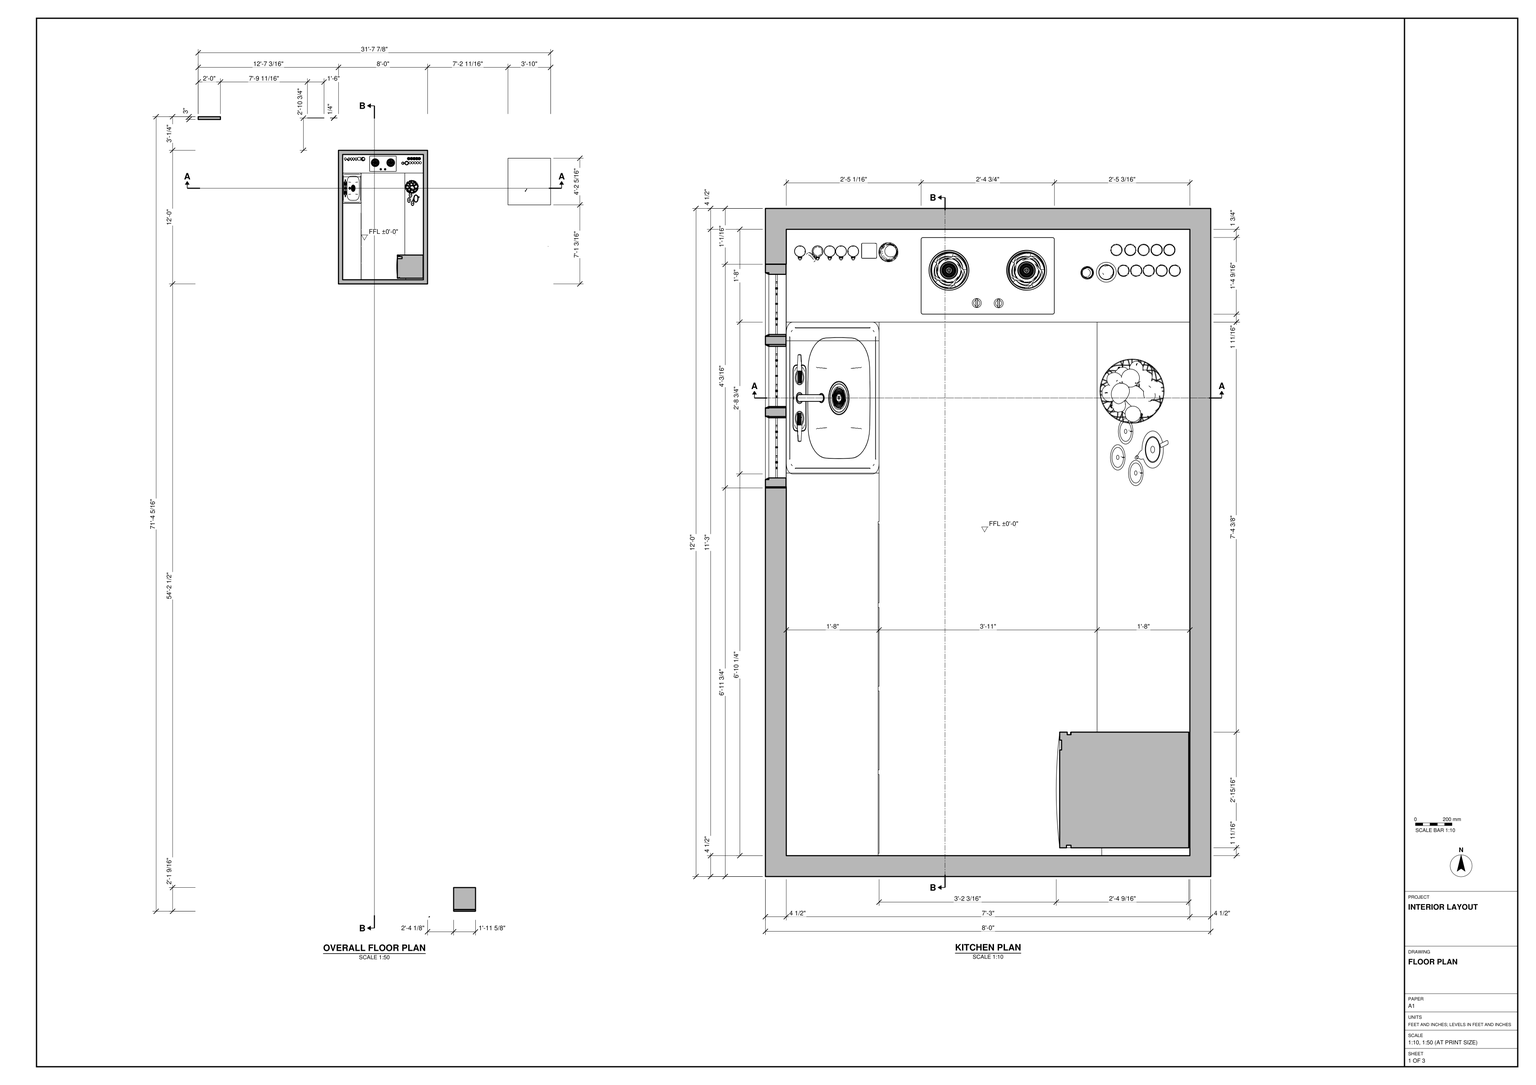
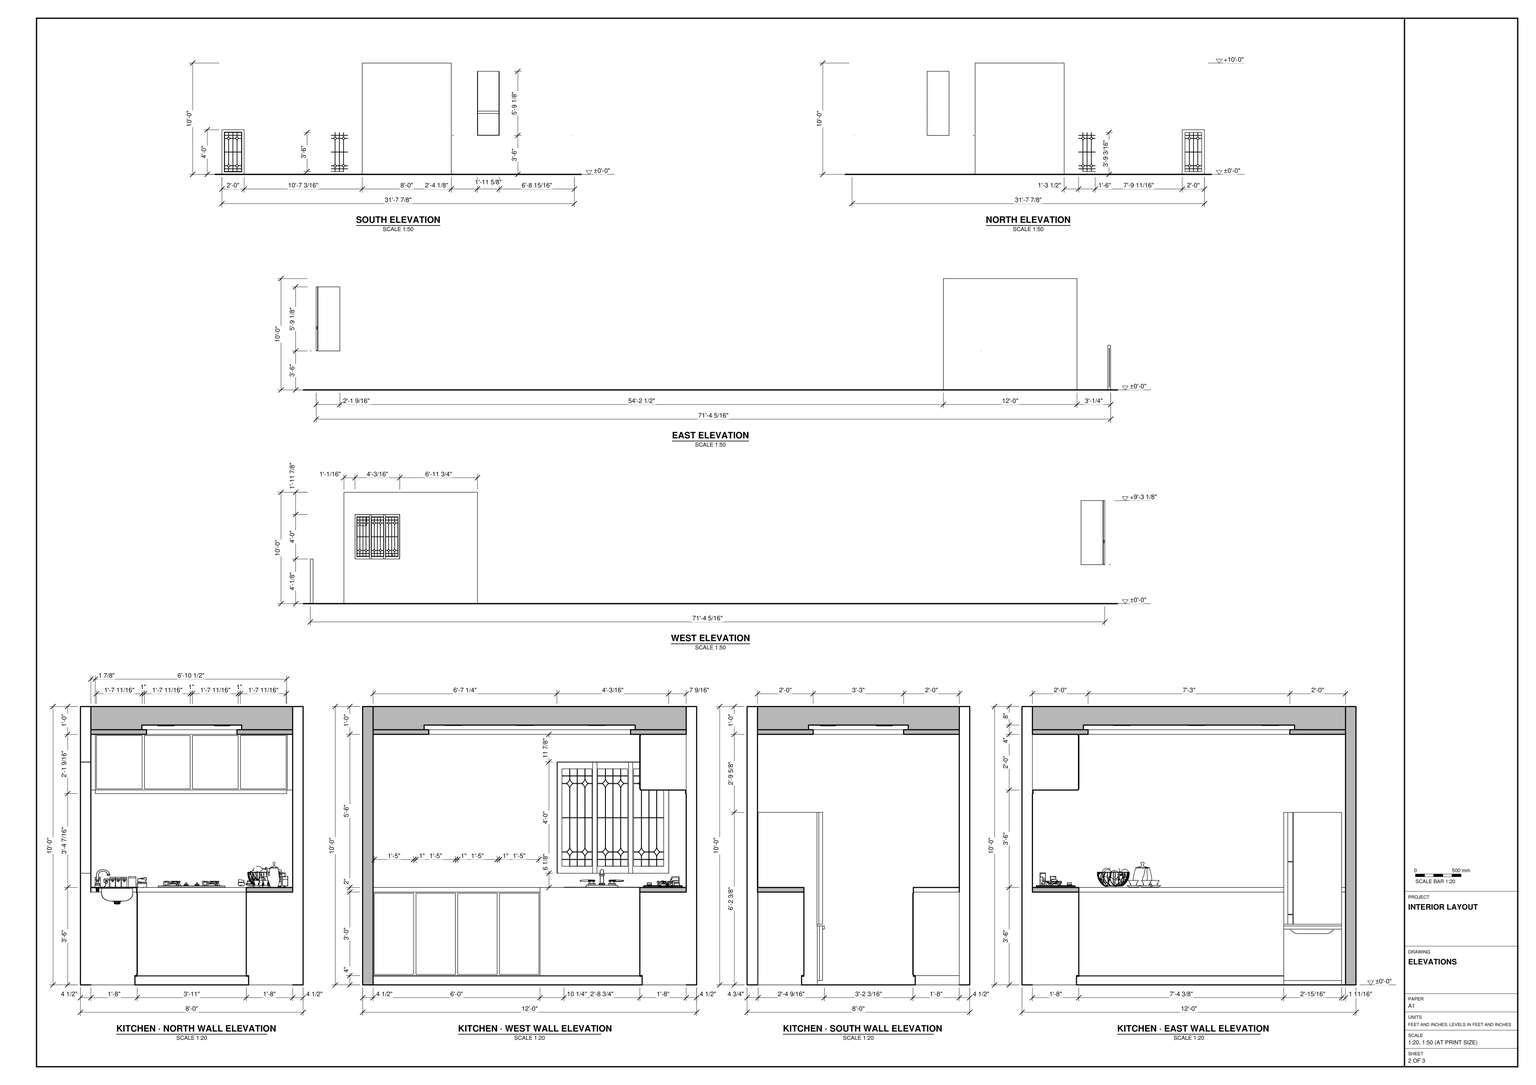
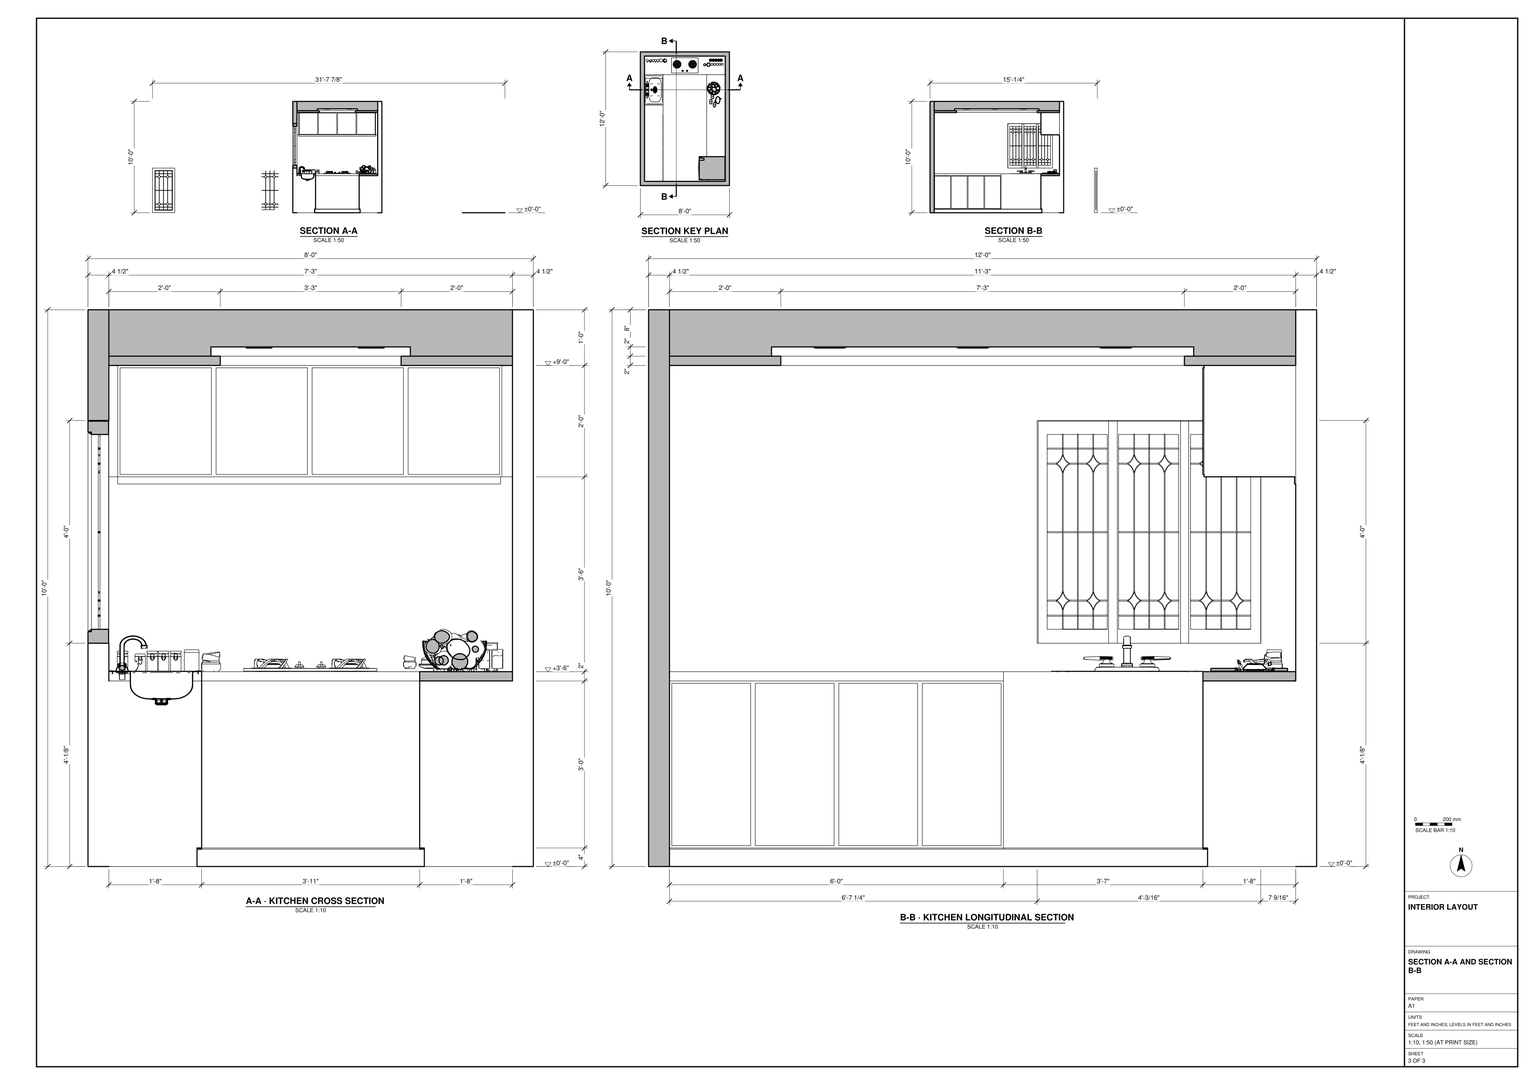
Build the kitchen in SketchUp from task_files/diagram_01.pdf. Work in feet and inches, with the finished floor at ±0'-0". Use the overall plan and elevations to position the kitchen and the detached elements outside it. The complete layout is 31'-7 7/8" wide by 71'-4 5/16" long and 10'-0" high; these are not the dimensions of the kitchen itself.

Model the kitchen shell at 8'-0" by 12'-0" externally, with 4 1/2" perimeter walls. Use the sections to form the floor and the stepped ceiling with its recessed central field. Fit the worktops along the north, west and east walls, leaving the central aisle clear. Follow the interior elevations for the extent and front divisions of the west base cabinets and the north wall cabinets. Set the sink and tap beneath the divided west window, place the cooktop on the north worktop and fit the refrigerator at the south end of the east run. Place the small countertop items in the areas indicated on the kitchen plan. Appliances, decor and loose items may be any suitable library components.

Keep shell elements and individual furniture or joinery pieces in separate groups or components, and use components for repeated parts. Save one SketchUp model as output_files/kitchen_interior_and_its_dimensioned_overall_layout.skp.

# SketchUp Ruby script. Lengths in inches.
U = 1.inch
M = Sketchup.active_model
def pt(a) = Geom::Point3d.new(a.map { |v| v * U })
def face(e, loops, mat)
  f = e.add_face(loops[0].map { |a| pt(a) })
  loops[1..].each { |l| e.add_face(l.map { |a| pt(a) }).erase! }
  f.material = f.back_material = mat if mat
  f
end
# faces: each face lists its corners as indices into pts; further lists are holes
def faces(e, pts, list, mat = nil) = list.each { |f| face(e, (f[0].is_a?(Array) ? f : [f]).map { |l| l.map { |i| pts[i] } }, mat) }
# xy, xz, yz: faces in a plane at the given z, y or x. An outline is a flat list of corners, or four numbers for a rectangle; further outlines are holes
def ring(l) = l.size == 4 ? [[l[0], l[1]], [l[2], l[1]], [l[2], l[3]], [l[0], l[3]]] : l.each_slice(2).to_a
def flat(e, list, mat, &to3) = list.each { |f| face(e, (f[0].is_a?(Array) ? f : [f]).map { |l| ring(l).map { |u, v| to3.(u, v) } }, mat) }
def xy(e, z, list, mat = nil) = flat(e, list, mat) { |x, y| [x, y, z] }
def xz(e, y, list, mat = nil) = flat(e, list, mat) { |x, z| [x, y, z] }
def yz(e, x, list, mat = nil) = flat(e, list, mat) { |y, z| [x, y, z] }
def lines(e, pts, list) = list.each { |a, b| e.add_line(pt(pts[a]), pt(pts[b])) }
# prism: a flat outline (further loops are holes) pulled along v
def prism(e, loops, v, mat = nil)
  f = face(e, loops, mat); d = Geom::Vector3d.new(v.map { |x| x * U })
  f.pushpull(f.normal.samedirection?(d) ? d.length : -d.length)
end
def box(e, o, s, mat = nil) = prism(e, [[o, [o[0] + s[0], o[1], o[2]], [o[0] + s[0], o[1] + s[1], o[2]], [o[0], o[1] + s[1], o[2]]]], [0, 0, s[2]], mat)
def at(x, y, z, deg = 0) = Geom::Transformation.translation(pt([x, y, z])) * Geom::Transformation.rotation(ORIGIN, Z_AXIS, deg.degrees)
def axes(o, x, y, z) = Geom::Transformation.new([*x, 0, *y, 0, *z, 0, *pt(o).to_a, 1])
def part(name) = M.definitions.add(name)
# library, detail: a bought-in or finely detailed component or shape, given as its bounding box
def library(name, o, s) = part(name).tap { |d| box(d.entities, o, s) }
def detail(e, o, s) = box(e.add_group.entities, o, s)
def put(e, d, t, mat = nil) = e.add_instance(d, t).tap { |i| i.material = mat if mat }
def group(e, t, mat = nil) = e.add_group.tap { |g| g.transformation = t; g.material = mat if mat }.entities
root = M.entities
M.materials.add("YS_Metal_SS1").color = [228, 228, 228]
M.materials.add("[0010_Snow]").color = [255, 255, 255]
M.materials.add("[Cladding Siding Tan]").color = [170, 170, 170]
M.materials.add("[Color M09]").color = [0, 0, 0]
M.materials.add("[Color_A01]").color = [255, 0, 0]
M.materials.add("[Granite Dark Gray]").color = [69, 68, 68]
M.materials.add("[Translucent Glass Gray]").color = [128, 128, 128]
M.materials["[Translucent Glass Gray]"].alpha = 0.5
M.materials.add("[Wood Veneer 02]").color = [190, 128, 91]
M.materials.add("[Wood_ Floor]").color = [154, 105, 59]
M.materials.add("spaghetti_A1").color = [203, 118, 20]
c1 = library("SINK (1)",[22.9375,3.09,31.55],[14.875,14.88,14.9])
c2 = library("GasStove_Black",[0,0,0],[28.74,16.54,2.72])
c3 = library("Fruit+Bowl+2",[0,0,0],[14.72,14,9.31])
c4 = library("cup set",[0.62,0.62,0],[2.74,2.74,1.14])
c5 = library("Group\#2",[319.64,-186.13,316.33],[171.98,171.98,176.14])
c6 = library("Group\#3",[-252.59,-194.96,554.0625],[177.73,177.73,123.23])
c7 = library("Group\#4",[-391.77,-168.5,554.09],[114.48,114.48,114.77])
c8 = library("Group\#5",[165.5,-155.83,316.17],[135.52,135.54,195.73])
c9 = library("Group\#8",[-62.35,-144.07,554.28],[103.86,103.86,170.6])
c10 = library("Group\#9",[51.41,-144.07,554.28],[103.86,103.86,170.6])
c11 = library("Group\#10",[163.08,-144.02,554.28],[103.75,103.76,170.6])
c12 = library("Group\#11",[278.63,-144.07,554.28],[103.86,103.86,170.6])
c13 = library("Group\#12",[395.59,-144.07,554.28],[103.86,103.86,170.6])
c14 = library("Group\#13",[-328.66,-188.67,316.12],[151.64,146.26,158.64])
c15 = library("Group\#14",[-167.96,-170.65,316.14],[99.3,128.23,183.55])
c16 = library("Group\#15",[-67.08,-170.69,316.14],[99.29,128.27,183.55])
c17 = library("Group\#16",[41.58,-170.65,316.14],[99.27,128.23,183.55])
c18 = library("Group\#17",[-421.22,-144.07,-0.09],[103.86,103.86,260.39])
c19 = library("Group\#18",[-296.9375,-144.07,-0.09],[103.86,103.86,260.39])
c20 = library("Group\#19",[-178.14,-144.07,-0.09],[103.85,103.86,260.39])
c21 = library("Group\#20",[-61.59,-144.02,-0.09],[103.75,103.76,260.39])
c22 = library("Group\#21",[51.71,-144.07,-0.09],[103.86,103.86,260.39])
c23 = library("Group\#28",[-433.81,-170.65,316.14],[99.3,128.23,183.55])
c24 = library("Group5\#1",[-3,-2,0],[6.43,4,4.1])
c25 = library("Group6\#1",[-1,-0.13,0.02],[1.21,0.26,0.16])
c26 = library("Group\#146",[0,0,0],[60.64,55.48,158.625])
c27 = part("Kitchen layout")
xy(c27.entities,0,[[19,0,68,116],[68,0,87,26.625]])
xy(c27.entities,3.746,[[19,115,68,116]])
xy(c27.entities,3.75,[[19,0,19,115,20,115,20,72,19.8,72,19.8,0],[67,26.625,68,115]],"spaghetti_A1")
xy(c27.entities,4,[[19,0,19.8,0,19.8,72,20,72,20,115,19,115],[67,26.625,68,115],[19,115,68,116]])
xy(c27.entities,4.5,[[19.8,0.5,20,17.5],[19.8,18.5,20,35.5],[19.8,36.5,20,53.5],[19.8,54.5,20,71.5]])
xy(c27.entities,39.5,[[19.8,0.5,20,17.5],[19.8,18.5,20,35.5],[19.8,36.5,20,53.5],[19.8,54.5,20,71.5]])
xy(c27.entities,40,[[67,26.625,87,115],[0,115,87,135]])
xy(c27.entities,42,[[0,110.98,20,115]])
xy(c27.entities,42,[[0,0,19.8,0,19.8,72,20,72,20,82.46,0,82.46],[67,26.625,87,115],[0,115,87,135]],"[Granite Dark Gray]")
xy(c27.entities,82.45,[[1.906,134.75,84.428,135]])
xy(c27.entities,84,[[1.906,115.25,1.906,134.75,84.428,134.75,84.428,135,84.709,135,84.709,115.25]])
xy(c27.entities,84.5,[[2.406,115,22.107,115.25],[23.107,115,42.808,115.25],[43.808,115,63.508,115.25],[64.508,115,84.209,115.25]])
xy(c27.entities,107.5,[[2.406,115,22.107,115.25],[23.107,115,42.808,115.25],[43.808,115,63.508,115.25],[64.508,115,84.209,115.25]])
xy(c27.entities,108,[[1.906,115.25,84.709,135]])
xz(c27.entities,0,[[19,3.75,19.8,4]])
xz(c27.entities,0,[[0,40,19.8,42]],"[Granite Dark Gray]")
xz(c27.entities,0,[[0,0,19,4],[0,4,19.8,40]],"[Wood Veneer 02]")
xz(c27.entities,0.5,[[19.8,4.5,20,39.5]])
xz(c27.entities,17.5,[[19.8,4.5,20,39.5]])
xz(c27.entities,18.5,[[19.8,4.5,20,39.5]])
xz(c27.entities,26.625,[[68,0,87,0,87,40,67,40,67,4,68,4],[67,3.75,68,4],[67,40,87,42]])
xz(c27.entities,35.5,[[19.8,4.5,20,39.5]])
xz(c27.entities,36.5,[[19.8,4.5,20,39.5]])
xz(c27.entities,53.5,[[19.8,4.5,20,39.5]])
xz(c27.entities,54.5,[[19.8,4.5,20,39.5]])
xz(c27.entities,71.5,[[19.8,4.5,20,39.5]])
xz(c27.entities,72,[[19.8,3.75,20,4],[19.8,4,20,40],[19.8,40,20,42]])
xz(c27.entities,115,[[19,3.746,20,3.75],[67,3.746,68,3.75],[19,3.75,20,4],[67,3.75,68,4],[20,4,67,40],
  [0,40,20,42],[67,40,87,42]])
xz(c27.entities,115,[[20,40,67,42]],"[Granite Dark Gray]")
xz(c27.entities,115,[[2.406,84.5,22.107,107.5],[23.107,84.5,42.808,107.5],[43.808,84.5,63.508,107.5],[64.508,84.5,84.209,107.5]],"[Translucent Glass Gray]")
xz(c27.entities,115,[[20,3.746,67,4]],"spaghetti_A1")
xz(c27.entities,115.25,[[[1.906,84,84.709,108],[23.107,84.5,42.808,107.5],[43.808,84.5,63.508,107.5],[2.406,84.5,22.107,107.5],[64.508,84.5,84.209,107.5]]],"[Color M09]")
xz(c27.entities,116,[[19,0,68,3.746],[19,3.746,68,4]])
xz(c27.entities,134.75,[[1.906,82.45,84.428,84]],"spaghetti_A1")
xz(c27.entities,135,[[0,40,87,42],[0,42,87,42,87,84,84.428,84,84.428,82.45,1.906,82.45,1.906,84,0,84],[0,84,1.906,108],[84.709,84,87,108],[0,108,87,120]])
yz(c27.entities,0,[[0,40,115,42],[115,40,135,42],[[0,42,135,120],[79.5,48.13,127.5,96]]])
yz(c27.entities,1.906,[[134.75,82.45,135,84],[115.25,84,135,108]])
yz(c27.entities,2.406,[[115,84.5,115.25,107.5]])
yz(c27.entities,19,[[115,3.746,116,4],[0,3.75,115,4]])
yz(c27.entities,19,[[0,0,116,0,116,3.746,115,3.746,115,3.75,0,3.75]],"[Wood Veneer 02]")
yz(c27.entities,19.8,[[0,3.75,72,4],[[0,4,72,40],[0.5,4.5,17.5,39.5],[18.5,4.5,35.5,39.5],[36.5,4.5,53.5,39.5],[54.5,4.5,71.5,39.5]]])
yz(c27.entities,19.8,[[0,40,72,42]],"[Granite Dark Gray]")
yz(c27.entities,20,[[72,3.75,115,4],[72,4,115,42]])
yz(c27.entities,20,[[0.5,4.5,17.5,39.5],[18.5,4.5,35.5,39.5],[36.5,4.5,53.5,39.5],[54.5,4.5,71.5,39.5]],"[Wood Veneer 02]")
yz(c27.entities,22.107,[[115,84.5,115.25,107.5]])
yz(c27.entities,23.107,[[115,84.5,115.25,107.5]])
yz(c27.entities,42.808,[[115,84.5,115.25,107.5]])
yz(c27.entities,43.808,[[115,84.5,115.25,107.5]])
yz(c27.entities,63.508,[[115,84.5,115.25,107.5]])
yz(c27.entities,64.508,[[115,84.5,115.25,107.5]])
yz(c27.entities,67,[[26.625,3.75,115,4],[26.625,4,115,40]])
yz(c27.entities,67,[[26.625,40,115,42]],"[Granite Dark Gray]")
yz(c27.entities,68,[[26.625,0,116,0,116,3.746,115,3.746,115,3.75,26.625,3.75],[115,3.746,116,4],[26.625,3.75,115,4]])
yz(c27.entities,84.209,[[115,84.5,115.25,107.5]])
yz(c27.entities,84.428,[[134.75,82.45,135,84]])
yz(c27.entities,84.709,[[115.25,84,135,108]])
yz(c27.entities,87,[[0,0,26.625,40],[0,40,26.625,42],[26.625,40,115,42],[115,40,135,42],[0,42,135,120]])
p = [[221.417,35.98,41.915],[221.441,35.98,41.915],[221.441,36.004,41.915],[92.685,-686.89,42],[93.685,-686.89,42],[93.685,-685.89,42]]
lines(c27.entities,p,[[0,1],[1,2],[2,0],[3,4],[4,5],[5,3]])
put(c27.entities,c1,axes([24.16,31.82,3.24],[0,2.1999,0],[-1.34454,0,0],[0,0,1]))
put(c27.entities,c2,at(29.05,116.71,42))
put(c27.entities,c3,at(67,93.1875,42))
put(c27.entities,c4,axes([69.17,81.87,42],[1.15,0,0],[0,2,0],[0,0,2.66351]))
put(c27.entities,c4,axes([70.87,87.48,42],[1.15,0,0],[0,2,0],[0,0,2.66351]),"[Color_A01]")
put(c27.entities,c4,axes([73.05,78.51,42],[1.15,0,0],[0,2,0],[0,0,2.66351]))
put(c27.entities,c5,axes([12.22,132.49,34.37],[0.02413,0,0],[0,0.02413,0],[0,0,0.02413]))
put(c27.entities,c6,axes([72.9375,128.3125,29.31],[0.02413,0,0],[0,0.02413,0],[0,0,0.02413]))
put(c27.entities,c7,axes([72.9375,128.3125,29.31],[0.02413,0,0],[0,0.02413,0],[0,0,0.02413]))
put(c27.entities,c8,axes([12.22,132.49,34.37],[0.02413,0,0],[0,0.02413,0],[0,0,0.02413]))
put(c27.entities,c9,axes([72.9375,128.3125,29.31],[0.02413,0,0],[0,0.02413,0],[0,0,0.02413]))
put(c27.entities,c10,axes([72.9375,128.3125,29.31],[0.02413,0,0],[0,0.02413,0],[0,0,0.02413]))
put(c27.entities,c11,axes([72.9375,128.3125,29.31],[0.02413,0,0],[0,0.02413,0],[0,0,0.02413]))
put(c27.entities,c12,axes([72.9375,128.3125,29.31],[0.02413,0,0],[0,0.02413,0],[0,0,0.02413]))
put(c27.entities,c13,axes([72.9375,128.3125,29.31],[0.02413,0,0],[0,0.02413,0],[0,0,0.02413]))
put(c27.entities,c14,axes([12.22,132.49,34.37],[0.02413,0,0],[0,0.02413,0],[0,0,0.02413]))
put(c27.entities,c15,axes([12.22,132.49,34.37],[0.02413,0,0],[0,0.02413,0],[0,0,0.02413]))
put(c27.entities,c16,axes([12.22,132.49,34.37],[0.02413,0,0],[0,0.02413,0],[0,0,0.02413]))
put(c27.entities,c17,axes([12.22,132.49,34.37],[0.02413,0,0],[0,0.02413,0],[0,0,0.02413]))
put(c27.entities,c18,axes([80.07,132.78,42],[0.02413,0,0],[0,0.02413,0],[0,0,0.02413]))
put(c27.entities,c19,axes([80.07,132.78,42],[0.02413,0,0],[0,0.02413,0],[0,0,0.02413]))
put(c27.entities,c20,axes([80.07,132.78,42],[0.02413,0,0],[0,0.02413,0],[0,0,0.02413]))
put(c27.entities,c21,axes([80.07,132.78,42],[0.02413,0,0],[0,0.02413,0],[0,0,0.02413]))
put(c27.entities,c22,axes([80.07,132.78,42],[0.02413,0,0],[0,0.02413,0],[0,0,0.02413]))
put(c27.entities,c23,axes([12.22,132.49,34.37],[0.02413,0,0],[0,0.02413,0],[0,0,0.02413]))
g1 = group(c27.entities,at(178.19,80.66,0),"[Wood_ Floor]")
xy(g1,0,[[0,0,45.97,50.31]])
put(c27.entities,c24,axes([78.98,87.53,42.01],[-1.10741,-0.53925,0],[0.31007,-1.92593,0],[0,0,2.66351]),"[0010_Snow]")
put(c27.entities,c25,axes([197.05,95.64,-0.04],[-1.49172,-2.29834,0],[2.29834,-1.49172,0],[0,0,2.74]),"[0010_Snow]")
put(c27.entities,c26,axes([58.1875,26.625,0],[0,-0.4111,0],[0.515,0,0],[0,0,0.46877]))
g2 = group(c27.entities,at(119.6,-680.6,42))
box(g2,[0,1.97,0],[23.62,23.62,69.09],"YS_Metal_SS1")
p = [[0,0,0],[1,0,0],[1,1,0]]
lines(g2,p,[[0,1],[1,2],[2,0]])
g3 = group(g2,at(0,0,0))
xy(g3,0.28,[[0.39,0,0.29,0.01,0.2,0.05,0.12,0.12,0.05,0.2,0.01,0.29,0,0.39,0,1.57,23.62,1.57,23.62,0.39,23.61,0.29,23.57,0.2,23.51,0.12,23.43,0.05,23.33,0.01,23.23,0]],"[Cladding Siding Tan]")
xy(g3,23.62,[[0.39,0,23.23,0,23.33,0.01,23.43,0.05,23.51,0.12,23.57,0.2,23.61,0.29,23.62,0.39,23.62,0.79,0,0.79,0,0.39,0.01,0.29,0.05,0.2,0.12,0.12,0.2,0.05,0.29,0.01],[0,0.79,23.62,1.57]],"[Cladding Siding Tan]")
xy(g3,26.2,[[0.39,0,0.29,0.01,0.2,0.05,0.12,0.12,0.05,0.2,0.01,0.29,0,0.39,0,0.79,23.62,0.79,23.62,0.39,23.61,0.29,23.57,0.2,23.51,0.12,23.43,0.05,23.33,0.01,23.23,0],[0,0.79,23.62,1.57]],"[Cladding Siding Tan]")
xy(g3,69.09,[[0.39,0,23.23,0,23.33,0.01,23.43,0.05,23.51,0.12,23.57,0.2,23.61,0.29,23.62,0.39,23.62,1.57,0,1.57,0,0.39,0.01,0.29,0.05,0.2,0.12,0.12,0.2,0.05,0.29,0.01]],"[Cladding Siding Tan]")
xz(g3,0,[[0.39,0.28,23.23,23.62],[0.39,26.2,23.23,69.09]],"[Cladding Siding Tan]")
xz(g3,0.79,[[0,23.62,23.62,26.2]],"[Cladding Siding Tan]")
xz(g3,1.57,[[0,0.28,23.62,23.62],[0,23.62,23.62,26.2],[0,26.2,23.62,69.09]],"[Cladding Siding Tan]")
yz(g3,0,[[0.39,0.28,1.57,23.62],[0.39,26.2,1.57,69.09]],"YS_Metal_SS1")
yz(g3,0,[[0.79,23.62,1.57,26.2]],"[Cladding Siding Tan]")
yz(g3,23.62,[[0.39,0.28,1.57,23.62],[0.39,26.2,1.57,69.09]],"YS_Metal_SS1")
yz(g3,23.62,[[0.79,23.62,1.57,26.2]],"[Cladding Siding Tan]")
p = [[0.29,0.01,0.28],[0.29,0.01,23.62],[0.2,0.05,23.62],[0.2,0.05,0.28],[0.39,0,0.28],[0.39,0,23.62],
  [23.23,0,23.62],[23.23,0,0.28],[23.33,0.01,0.28],[23.33,0.01,23.62],[23.43,0.05,0.28],[23.43,0.05,23.62],
  [0.12,0.12,23.62],[0.12,0.12,0.28],[0.05,0.2,23.62],[0.05,0.2,0.28],[23.51,0.12,0.28],[23.51,0.12,23.62],
  [23.57,0.2,0.28],[23.57,0.2,23.62],[0.01,0.29,23.62],[0.01,0.29,0.28],[23.61,0.29,0.28],[23.61,0.29,23.62],
  [0,0.39,23.62],[0,0.39,0.28],[23.62,0.39,0.28],[23.62,0.39,23.62],[0.29,0.01,26.2],[0.29,0.01,69.09],
  [0.2,0.05,69.09],[0.2,0.05,26.2],[0.39,0,26.2],[0.39,0,69.09],[23.23,0,69.09],[23.23,0,26.2],
  [23.33,0.01,26.2],[23.33,0.01,69.09],[23.43,0.05,26.2],[23.43,0.05,69.09],[0.12,0.12,69.09],[0.12,0.12,26.2],
  [0.05,0.2,69.09],[0.05,0.2,26.2],[23.51,0.12,26.2],[23.51,0.12,69.09],[23.57,0.2,26.2],[23.57,0.2,69.09],
  [0.01,0.29,69.09],[0.01,0.29,26.2],[23.61,0.29,26.2],[23.61,0.29,69.09],[0,0.39,69.09],[0,0.39,26.2],
  [23.62,0.39,26.2],[23.62,0.39,69.09]]
faces(g3,p,[[0,1,2,3],[4,5,1,0],[6,7,8,9],[9,8,10,11],[3,2,12,13],[13,12,14,15],[11,10,16,17],[17,16,18,19],
  [15,14,20,21],[19,18,22,23],[21,20,24,25],[23,22,26,27],[28,29,30,31],[32,33,29,28],[34,35,36,37],[37,36,38,39],
  [31,30,40,41],[41,40,42,43],[39,38,44,45],[45,44,46,47],[43,42,48,49],[47,46,50,51],[49,48,52,53],[51,50,54,55]],"YS_Metal_SS1")
lines(g3,p,[[32,5],[6,35]])
c28 = library("grill",[0,0,0],[18,0.25,42])
c29 = library("Window sash",[0,0,0],[24,3,48])
c30 = library("window3",[0,0,0],[66.9375,3,48])
xy(root,-0.13,[[[0,676.1,96,820.1],[4.5,680.6,91.5,815.6]]])
xy(root,48,[[0,760.1,4.5,808.1]])
xy(root,95.87,[[0,760.1,4.5,808.1]])
xy(root,119.87,[[[0,676.1,96,820.1],[4.5,680.6,91.5,815.6]]])
xz(root,676.1,[[0,-0.13,96,119.87]])
xz(root,680.6,[[4.5,-0.13,91.5,119.87]])
xz(root,760.1,[[0,48,4.5,95.87]])
xz(root,808.1,[[0,48,4.5,95.87]])
xz(root,820.1,[[0,-0.13,96,119.87]])
yz(root,0,[[[676.1,-0.13,820.1,119.87],[760.1,48,808.1,95.87]]])
yz(root,96,[[676.1,-0.13,820.1,119.87]])
put(root,c27,at(4.5,680.6,-0.13))
put(root,c28,at(-33.51,854.82,3.0625))
put(root,c29,at(-151.21,853.32,0))
put(root,c30,axes([0,808.06,48],[0,-0.72,0],[1.48075,0,0],[0,0,1]))
g4 = group(root,at(4.5,680.6,119.87))
xy(g4,-12,[[[0,0,87,135],[24,24,63,111]]])
xy(g4,-10,[[[0,0,87,135],[22,22,65,113]],[22,22,24,111],[24,22,63,24],[63,22,65,111],[22,111,65,113]])
xy(g4,-8,[[22,22,65,113]])
xy(g4,0,[[0,0,87,135]])
xz(g4,0,[[0,-12,87,-10],[0,-10,87,0]])
xz(g4,22,[[22,-10,65,-8]],"spaghetti_A1")
xz(g4,24,[[24,-12,63,-10]])
xz(g4,111,[[24,-12,63,-10]])
xz(g4,113,[[22,-10,65,-8]],"spaghetti_A1")
xz(g4,135,[[0,-12,87,-10],[0,-10,87,0]])
yz(g4,0,[[0,-12,135,-10],[0,-10,135,0]])
yz(g4,22,[[22,-10,113,-8]],"spaghetti_A1")
yz(g4,24,[[24,-12,111,-10]])
yz(g4,63,[[24,-12,111,-10]])
yz(g4,65,[[22,-10,113,-8]],"spaghetti_A1")
yz(g4,87,[[0,-12,135,-10],[0,-10,135,0]])
g5 = group(g4,at(52.89,28.89,-8),"spaghetti_A1")
prism(g5,[[[5.02,7.09,-0.25],[4.09,7.33,-0.25],[3.125,7.3125,-0.25],[2.2,7.05,-0.25],[1.375,6.55,-0.25],[0.7,5.86,-0.25],[0.23,5.02,-0.25],[0,4.09,-0.25],[0.01,3.125,-0.25],[0.28,2.2,-0.25],[0.77,1.375,-0.25],[1.46,0.7,-0.25],[2.3,0.23,-0.25],[3.24,0,-0.25],[4.2,0.01,-0.25],[5.125,0.28,-0.25],[5.95,0.77,-0.25],[6.62,1.46,-0.25],[7.09,2.3,-0.25],[7.33,3.24,-0.25],[7.3125,4.2,-0.25],[7.05,5.125,-0.25],[6.55,5.95,-0.25],[5.86,6.62,-0.25]]],[0,0,0.25])
xy(g5,-0.25,[[-20.95,2,-19.99,2.01,-19.0625,2.28,-18.24,2.77,-17.57,3.46,-17.1,4.3,-16.86,5.24,-16.875,6.2,-17.14,7.125,-17.63,7.95,-18.32,8.62,-19.17,9.09,-20.1,9.33,-21.0625,9.3125,-21.99,9.05,-22.8125,8.55,-23.48,7.86,-23.95,7.02,-24.1875,6.09,-24.17,5.125,-23.91,4.2,-23.42,3.375,-22.72,2.7,-21.88,2.23],[3.24,31.84,4.2,31.86,5.125,32.12,5.95,32.62,6.62,33.31,7.09,34.15,7.33,35.08,7.3125,36.04,7.05,36.97,6.55,37.8,5.86,38.47,5.02,38.93,4.09,39.17,3.125,39.15,2.2,38.89,1.375,38.4,0.7,37.71,0.23,36.87,0,35.93,0.01,34.97,0.28,34.04,0.77,33.22,1.46,32.55,2.3,32.08],[-20.95,32.84,-19.99,32.86,-19.0625,33.12,-18.24,33.62,-17.57,34.31,-17.1,35.15,-16.86,36.08,-16.875,37.04,-17.14,37.97,-17.63,38.8,-18.32,39.47,-19.17,39.93,-20.1,40.17,-21.0625,40.15,-21.99,39.89,-22.8125,39.4,-23.48,38.71,-23.95,37.87,-24.1875,36.93,-24.17,35.97,-23.91,35.04,-23.42,34.22,-22.72,33.55,-21.88,33.08],[-20.95,63.6875,-19.99,63.7,-19.0625,63.97,-18.24,64.46,-17.57,65.15,-17.1,65.99,-16.86,66.93,-16.875,67.89,-17.14,68.8125,-17.63,69.64,-18.32,70.31,-19.17,70.78,-20.1,71.01,-21.0625,71,-21.99,70.74,-22.8125,70.24,-23.48,69.55,-23.95,68.71,-24.1875,67.78,-24.17,66.8125,-23.91,65.89,-23.42,65.0625,-22.72,64.39,-21.88,63.92],[3.24,63.6875,4.2,63.7,5.125,63.97,5.95,64.46,6.62,65.15,7.09,65.99,7.33,66.93,7.3125,67.89,7.05,68.8125,6.55,69.64,5.86,70.31,5.02,70.78,4.09,71.01,3.125,71,2.2,70.74,1.375,70.24,0.7,69.55,0.23,68.71,0,67.78,0.01,66.8125,0.28,65.89,0.77,65.0625,1.46,64.39,2.3,63.92]])
p = [[4.09,39.17,0],[5.02,38.93,0],[2.2,38.89,0],[3.125,39.15,0],[5.86,38.47,0],[6.55,37.8,0],
  [7.05,36.97,0],[7.3125,36.04,0],[7.33,35.08,0],[7.09,34.15,0],[6.62,33.31,0],[5.95,32.62,0],
  [5.125,32.12,0],[4.2,31.86,0],[3.24,31.84,0],[2.3,32.08,0],[1.46,32.55,0],[0.77,33.22,0],
  [0.28,34.04,0],[0.01,34.97,0],[0,35.93,0],[0.23,36.87,0],[0.7,37.71,0],[1.375,38.4,0],
  [4.09,71.01,0],[5.02,70.78,0],[2.2,70.74,0],[3.125,71,0],[5.86,70.31,0],[6.55,69.64,0],
  [7.05,68.8125,0],[7.3125,67.89,0],[7.33,66.93,0],[7.09,65.99,0],[6.62,65.15,0],[5.95,64.46,0],
  [5.125,63.97,0],[4.2,63.7,0],[3.24,63.6875,0],[2.3,63.92,0],[1.46,64.39,0],[0.77,65.0625,0],
  [0.28,65.89,0],[0.01,66.8125,0],[0,67.78,0],[0.23,68.71,0],[0.7,69.55,0],[1.375,70.24,0],
  [-23.42,65.0625,0],[-23.91,65.89,0],[-21.99,70.74,0],[-21.0625,71,0],[-20.1,71.01,0],[-19.17,70.78,0],
  [-18.32,70.31,0],[-17.63,69.64,0],[-17.14,68.8125,0],[-16.875,67.89,0],[-16.86,66.93,0],[-17.1,65.99,0],
  [-17.57,65.15,0],[-18.24,64.46,0],[-19.0625,63.97,0],[-19.99,63.7,0],[-20.95,63.6875,0],[-21.88,63.92,0],
  [-22.72,64.39,0],[-24.17,66.8125,0],[-24.1875,67.78,0],[-23.95,68.71,0],[-23.48,69.55,0],[-22.8125,70.24,0],
  [-18.24,33.62,0],[-19.0625,33.12,0],[-21.99,39.89,0],[-21.0625,40.15,0],[-20.1,40.17,0],[-19.17,39.93,0],
  [-18.32,39.47,0],[-17.63,38.8,0],[-17.14,37.97,0],[-16.875,37.04,0],[-16.86,36.08,0],[-17.1,35.15,0],
  [-17.57,34.31,0],[-19.99,32.86,0],[-20.95,32.84,0],[-21.88,33.08,0],[-22.72,33.55,0],[-23.42,34.22,0],
  [-23.91,35.04,0],[-24.17,35.97,0],[-24.1875,36.93,0],[-23.95,37.87,0],[-23.48,38.71,0],[-22.8125,39.4,0],
  [-18.24,2.77,0],[-19.0625,2.28,0],[-21.99,9.05,0],[-21.0625,9.3125,0],[-20.1,9.33,0],[-19.17,9.09,0],
  [-18.32,8.62,0],[-17.63,7.95,0],[-17.14,7.125,0],[-16.875,6.2,0],[-16.86,5.24,0],[-17.1,4.3,0],
  [-17.57,3.46,0],[-19.99,2.01,0],[-20.95,2,0],[-21.88,2.23,0],[-22.72,2.7,0],[-23.42,3.375,0],
  [-23.91,4.2,0],[-24.17,5.125,0],[-24.1875,6.09,0],[-23.95,7.02,0],[-23.48,7.86,0],[-22.8125,8.55,0]]
lines(g5,p,[[0,1],[2,3],[3,0],[1,4],[4,5],[5,6],[6,7],[7,8],[8,9],[9,10],[10,11],[11,12],
  [12,13],[13,14],[14,15],[15,16],[16,17],[17,18],[18,19],[19,20],[20,21],[21,22],[22,23],[23,2],
  [24,25],[26,27],[27,24],[25,28],[28,29],[29,30],[30,31],[31,32],[32,33],[33,34],[34,35],[35,36],
  [36,37],[37,38],[38,39],[39,40],[40,41],[41,42],[42,43],[43,44],[44,45],[45,46],[46,47],[47,26],
  [48,49],[50,51],[51,52],[52,53],[53,54],[54,55],[55,56],[56,57],[57,58],[58,59],[59,60],[60,61],
  [61,62],[62,63],[63,64],[64,65],[65,66],[66,48],[49,67],[67,68],[68,69],[69,70],[70,71],[71,50],
  [72,73],[74,75],[75,76],[76,77],[77,78],[78,79],[79,80],[80,81],[81,82],[82,83],[83,84],[84,72],
  [73,85],[85,86],[86,87],[87,88],[88,89],[89,90],[90,91],[91,92],[92,93],[93,94],[94,95],[95,74],
  [96,97],[98,99],[99,100],[100,101],[101,102],[102,103],[103,104],[104,105],[105,106],[106,107],[107,108],[108,96],
  [97,109],[109,110],[110,111],[111,112],[112,113],[113,114],[114,115],[115,116],[116,117],[117,118],[118,119],[119,98]])
